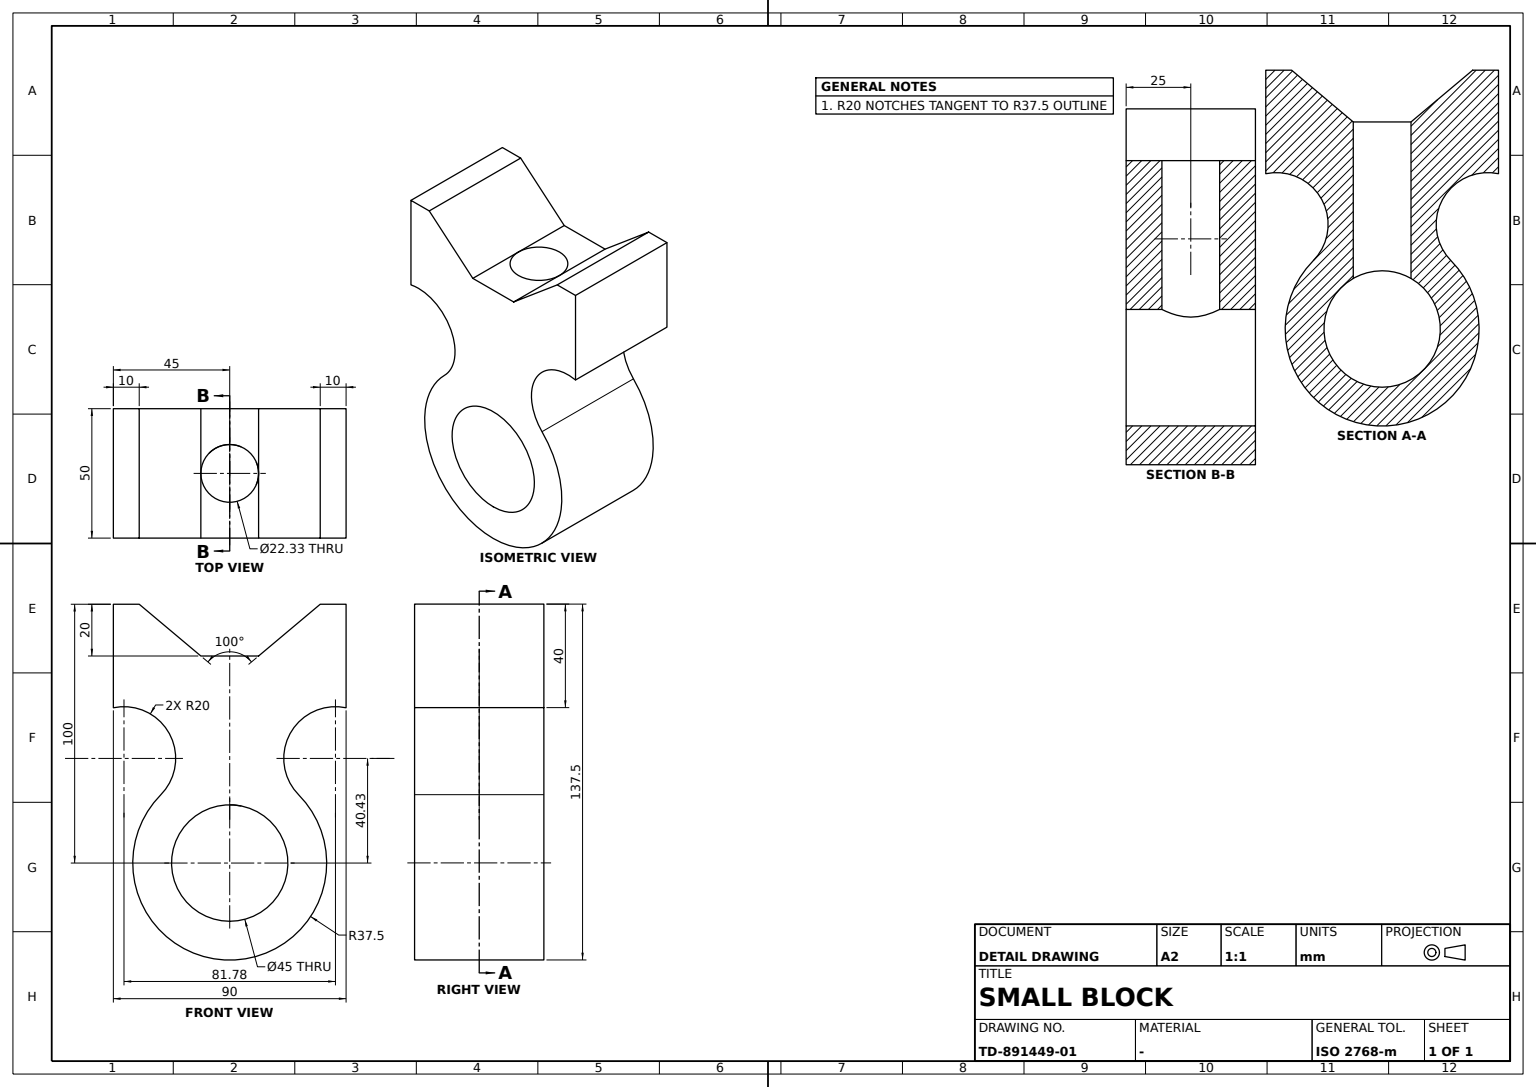
ISO-10303-21;
HEADER;
FILE_DESCRIPTION((''),'2;1');
FILE_NAME('','',(''),(''),'','','');
FILE_SCHEMA(('AUTOMOTIVE_DESIGN'));
ENDSEC;
DATA;
#1=APPLICATION_CONTEXT('');
#2=PRODUCT_CONTEXT('',#1,'mechanical');
#3=PRODUCT('','','',(#2));
#4=PRODUCT_DEFINITION_FORMATION('','',#3);
#5=PRODUCT_DEFINITION_CONTEXT('',#1,'design');
#6=PRODUCT_DEFINITION('','',#4,#5);
#7=PRODUCT_DEFINITION_SHAPE('','',#6);
#8=(LENGTH_UNIT()NAMED_UNIT(*)SI_UNIT(.MILLI.,.METRE.));
#9=(NAMED_UNIT(*)PLANE_ANGLE_UNIT()SI_UNIT($,.RADIAN.));
#10=(NAMED_UNIT(*)SI_UNIT($,.STERADIAN.)SOLID_ANGLE_UNIT());
#11=UNCERTAINTY_MEASURE_WITH_UNIT(LENGTH_MEASURE(0.005),#8,'distance_accuracy_value','');
#12=(GEOMETRIC_REPRESENTATION_CONTEXT(3)GLOBAL_UNCERTAINTY_ASSIGNED_CONTEXT((#11))GLOBAL_UNIT_ASSIGNED_CONTEXT((#8,#9,#10))REPRESENTATION_CONTEXT('',''));
#13=CARTESIAN_POINT('',(0.,-11.164928,80.));
#14=VERTEX_POINT('',#13);
#15=CARTESIAN_POINT('',(0.,11.164928,80.));
#16=VERTEX_POINT('',#15);
#17=CARTESIAN_POINT('',(0.,0.,80.));
#18=DIRECTION('',(0.,0.,-1.));
#19=DIRECTION('',(-1.,0.,0.));
#20=AXIS2_PLACEMENT_3D('',#17,#18,#19);
#21=CIRCLE('',#20,11.164928);
#22=EDGE_CURVE('',#14,#16,#21,.F.);
#23=ORIENTED_EDGE('',*,*,#22,.F.);
#24=CARTESIAN_POINT('',(25.,-11.164928,80.));
#25=VERTEX_POINT('',#24);
#26=DIRECTION('',(1.,0.,0.));
#27=VECTOR('',#26,1000.);
#28=LINE('',#13,#27);
#29=EDGE_CURVE('',#14,#25,#28,.T.);
#30=ORIENTED_EDGE('',*,*,#29,.T.);
#31=CARTESIAN_POINT('',(25.,11.164928,80.));
#32=VERTEX_POINT('',#31);
#33=CARTESIAN_POINT('',(25.,0.,80.));
#34=DIRECTION('',(0.,1.,0.));
#35=VECTOR('',#34,1000.);
#36=LINE('',#33,#35);
#37=EDGE_CURVE('',#25,#32,#36,.T.);
#38=ORIENTED_EDGE('',*,*,#37,.T.);
#39=LINE('',#15,#27);
#40=EDGE_CURVE('',#16,#32,#39,.T.);
#41=ORIENTED_EDGE('',*,*,#40,.F.);
#42=EDGE_LOOP('',(#23,#30,#38,#41));
#43=FACE_BOUND('',#42,.T.);
#44=AXIS2_PLACEMENT_3D('',#13,#18,#34);
#45=PLANE('',#44);
#46=ADVANCED_FACE('',(#43),#45,.F.);
#47=CARTESIAN_POINT('',(25.,-45.,100.));
#48=VERTEX_POINT('',#47);
#49=CARTESIAN_POINT('',(25.,-35.,100.));
#50=VERTEX_POINT('',#49);
#51=CARTESIAN_POINT('',(25.,0.,100.));
#52=LINE('',#51,#35);
#53=EDGE_CURVE('',#48,#50,#52,.T.);
#54=ORIENTED_EDGE('',*,*,#53,.T.);
#55=CARTESIAN_POINT('',(-25.,-35.,100.));
#56=VERTEX_POINT('',#55);
#57=CARTESIAN_POINT('',(0.,-35.,100.));
#58=LINE('',#57,#27);
#59=EDGE_CURVE('',#56,#50,#58,.T.);
#60=ORIENTED_EDGE('',*,*,#59,.F.);
#61=CARTESIAN_POINT('',(-25.,-45.,100.));
#62=VERTEX_POINT('',#61);
#63=CARTESIAN_POINT('',(-25.,0.,100.));
#64=LINE('',#63,#35);
#65=EDGE_CURVE('',#62,#56,#64,.T.);
#66=ORIENTED_EDGE('',*,*,#65,.F.);
#67=CARTESIAN_POINT('',(0.,-45.,100.));
#68=LINE('',#67,#27);
#69=EDGE_CURVE('',#62,#48,#68,.T.);
#70=ORIENTED_EDGE('',*,*,#69,.T.);
#71=EDGE_LOOP('',(#54,#60,#66,#70));
#72=FACE_BOUND('',#71,.T.);
#73=CARTESIAN_POINT('',(0.,35.,100.));
#74=AXIS2_PLACEMENT_3D('',#73,#18,#34);
#75=PLANE('',#74);
#76=ADVANCED_FACE('',(#72),#75,.F.);
#77=CARTESIAN_POINT('',(-25.,35.,100.));
#78=VERTEX_POINT('',#77);
#79=CARTESIAN_POINT('',(25.,35.,100.));
#80=VERTEX_POINT('',#79);
#81=LINE('',#73,#27);
#82=EDGE_CURVE('',#78,#80,#81,.T.);
#83=ORIENTED_EDGE('',*,*,#82,.F.);
#84=CARTESIAN_POINT('',(-25.,11.164928,80.));
#85=VERTEX_POINT('',#84);
#86=CARTESIAN_POINT('',(-25.,-34.779231,41.448273));
#87=DIRECTION('',(0.,0.766044443,0.64278761));
#88=VECTOR('',#87,1000.);
#89=LINE('',#86,#88);
#90=EDGE_CURVE('',#85,#78,#89,.T.);
#91=ORIENTED_EDGE('',*,*,#90,.F.);
#92=EDGE_CURVE('',#85,#16,#39,.T.);
#93=ORIENTED_EDGE('',*,*,#92,.T.);
#94=ORIENTED_EDGE('',*,*,#40,.T.);
#95=CARTESIAN_POINT('',(25.,-34.779231,41.448273));
#96=LINE('',#95,#88);
#97=EDGE_CURVE('',#32,#80,#96,.T.);
#98=ORIENTED_EDGE('',*,*,#97,.T.);
#99=EDGE_LOOP('',(#83,#91,#93,#94,#98));
#100=FACE_BOUND('',#99,.T.);
#101=DIRECTION('',(0.,0.64278761,-0.766044443));
#102=AXIS2_PLACEMENT_3D('',#15,#101,#87);
#103=PLANE('',#102);
#104=ADVANCED_FACE('',(#100),#103,.F.);
#105=CARTESIAN_POINT('',(-25.,0.,-22.5));
#106=VERTEX_POINT('',#105);
#107=CARTESIAN_POINT('',(-25.,0.,0.));
#108=AXIS2_PLACEMENT_3D('',#107,#26,#18);
#109=CIRCLE('',#108,22.5);
#110=EDGE_CURVE('',#106,#106,#109,.T.);
#111=ORIENTED_EDGE('',*,*,#110,.T.);
#112=EDGE_LOOP('',(#111));
#113=FACE_BOUND('',#112,.T.);
#114=ORIENTED_EDGE('',*,*,#90,.T.);
#115=CARTESIAN_POINT('',(-25.,45.,100.));
#116=VERTEX_POINT('',#115);
#117=EDGE_CURVE('',#78,#116,#64,.T.);
#118=ORIENTED_EDGE('',*,*,#117,.T.);
#119=CARTESIAN_POINT('',(-25.,45.,60.));
#120=VERTEX_POINT('',#119);
#121=CARTESIAN_POINT('',(-25.,45.,0.));
#122=VECTOR('',#18,1000.);
#123=LINE('',#121,#122);
#124=EDGE_CURVE('',#116,#120,#123,.T.);
#125=ORIENTED_EDGE('',*,*,#124,.T.);
#126=CARTESIAN_POINT('',(-25.,26.666657,26.365496));
#127=VERTEX_POINT('',#126);
#128=CARTESIAN_POINT('',(-25.,40.888875,40.427094));
#129=AXIS2_PLACEMENT_3D('',#128,#26,#18);
#130=CIRCLE('',#129,20.);
#131=EDGE_CURVE('',#120,#127,#130,.T.);
#132=ORIENTED_EDGE('',*,*,#131,.T.);
#133=CARTESIAN_POINT('',(-25.,-26.666657,26.365496));
#134=VERTEX_POINT('',#133);
#135=CIRCLE('',#108,37.5);
#136=EDGE_CURVE('',#134,#127,#135,.T.);
#137=ORIENTED_EDGE('',*,*,#136,.F.);
#138=CARTESIAN_POINT('',(-25.,-45.,60.));
#139=VERTEX_POINT('',#138);
#140=CARTESIAN_POINT('',(-25.,-40.888875,40.427094));
#141=AXIS2_PLACEMENT_3D('',#140,#26,#18);
#142=CIRCLE('',#141,20.);
#143=EDGE_CURVE('',#134,#139,#142,.T.);
#144=ORIENTED_EDGE('',*,*,#143,.T.);
#145=CARTESIAN_POINT('',(-25.,-45.,0.));
#146=DIRECTION('',(0.,0.,1.));
#147=VECTOR('',#146,1000.);
#148=LINE('',#145,#147);
#149=EDGE_CURVE('',#139,#62,#148,.T.);
#150=ORIENTED_EDGE('',*,*,#149,.T.);
#151=ORIENTED_EDGE('',*,*,#65,.T.);
#152=CARTESIAN_POINT('',(-25.,-11.164928,80.));
#153=VERTEX_POINT('',#152);
#154=CARTESIAN_POINT('',(-25.,34.779231,41.448273));
#155=DIRECTION('',(0.,0.766044443,-0.64278761));
#156=VECTOR('',#155,1000.);
#157=LINE('',#154,#156);
#158=EDGE_CURVE('',#56,#153,#157,.T.);
#159=ORIENTED_EDGE('',*,*,#158,.T.);
#160=CARTESIAN_POINT('',(-25.,0.,80.));
#161=LINE('',#160,#35);
#162=EDGE_CURVE('',#153,#85,#161,.T.);
#163=ORIENTED_EDGE('',*,*,#162,.T.);
#164=EDGE_LOOP('',(#114,#118,#125,#132,#137,#144,#150,#151,#159,#163));
#165=FACE_BOUND('',#164,.T.);
#166=AXIS2_PLACEMENT_3D('',#107,#26,#34);
#167=PLANE('',#166);
#168=ADVANCED_FACE('',(#113,#165),#167,.F.);
#169=CARTESIAN_POINT('',(25.,34.779231,41.448273));
#170=LINE('',#169,#156);
#171=EDGE_CURVE('',#50,#25,#170,.T.);
#172=ORIENTED_EDGE('',*,*,#171,.T.);
#173=ORIENTED_EDGE('',*,*,#29,.F.);
#174=EDGE_CURVE('',#153,#14,#28,.T.);
#175=ORIENTED_EDGE('',*,*,#174,.F.);
#176=ORIENTED_EDGE('',*,*,#158,.F.);
#177=ORIENTED_EDGE('',*,*,#59,.T.);
#178=EDGE_LOOP('',(#172,#173,#175,#176,#177));
#179=FACE_BOUND('',#178,.T.);
#180=DIRECTION('',(0.,-0.64278761,-0.766044443));
#181=AXIS2_PLACEMENT_3D('',#57,#180,#155);
#182=PLANE('',#181);
#183=ADVANCED_FACE('',(#179),#182,.F.);
#184=CARTESIAN_POINT('',(25.,0.,-22.5));
#185=VERTEX_POINT('',#184);
#186=CARTESIAN_POINT('',(25.,0.,0.));
#187=AXIS2_PLACEMENT_3D('',#186,#26,#18);
#188=CIRCLE('',#187,22.5);
#189=EDGE_CURVE('',#185,#185,#188,.T.);
#190=ORIENTED_EDGE('',*,*,#189,.T.);
#191=EDGE_LOOP('',(#190));
#192=FACE_BOUND('',#191,.T.);
#193=ORIENTED_EDGE('',*,*,#110,.F.);
#194=EDGE_LOOP('',(#193));
#195=FACE_BOUND('',#194,.T.);
#196=CARTESIAN_POINT('',(-11.164928,0.,22.5));
#197=VERTEX_POINT('',#196);
#198=CARTESIAN_POINT('',(-10.549112,4.471728,22.185581));
#199=CARTESIAN_POINT('',(-11.471357,-0.004788,22.656475));
#200=CARTESIAN_POINT('',(-10.555027,-4.452577,22.188517));
#201=CARTESIAN_POINT('',(-8.083695,-8.096902,21.079337));
#202=CARTESIAN_POINT('',(-4.460245,-10.54731,19.903886));
#203=CARTESIAN_POINT('',(-0.033968,-11.469433,19.351981));
#204=CARTESIAN_POINT('',(4.433612,-10.564331,19.894948));
#205=CARTESIAN_POINT('',(8.071653,-8.106887,21.074896));
#206=CARTESIAN_POINT('',(10.544117,-4.481106,22.183139));
#207=CARTESIAN_POINT('',(11.471336,-0.0131,22.656464));
#208=CARTESIAN_POINT('',(10.560049,4.443068,22.190975));
#209=CARTESIAN_POINT('',(8.089148,8.091903,21.081417));
#210=CARTESIAN_POINT('',(4.463912,10.546318,19.904537));
#211=CARTESIAN_POINT('',(0.033992,11.469928,19.351655));
#212=CARTESIAN_POINT('',(-4.437338,10.56334,19.895601));
#213=CARTESIAN_POINT('',(-8.077104,8.101877,21.076977));
#214=B_SPLINE_CURVE_WITH_KNOTS('',3,(#198,#199,#200,#201,#202,#203,#204,#205,#206,#207,#208,#209,#210,#211,#212,#213,#198,#199,#200),.UNSPECIFIED.,.T.,.F.,(1,1,1,1,1,1,1,1,1,1,1,1,1,1,1,1,1,1,1,1,1,1,1),(-0.013302099,-0.008868066,-0.004434033,0.,0.004434033,0.008868066,0.013302099,0.017736132,0.022170165,0.026604198,0.031038231,0.035472264,0.039906297,0.04434033,0.048774363,0.053208396,0.057642429,0.062076462,0.066510495,0.070944528,0.075378561,0.079812594,0.084246628),.UNSPECIFIED.);
#215=EDGE_CURVE('',#197,#197,#214,.T.);
#216=ORIENTED_EDGE('',*,*,#215,.T.);
#217=EDGE_LOOP('',(#216));
#218=FACE_BOUND('',#217,.T.);
#219=CARTESIAN_POINT('',(0.,0.,0.));
#220=AXIS2_PLACEMENT_3D('',#219,#26,#34);
#221=CYLINDRICAL_SURFACE('',#220,22.5);
#222=ADVANCED_FACE('',(#192,#195,#218),#221,.F.);
#223=ORIENTED_EDGE('',*,*,#215,.F.);
#224=EDGE_LOOP('',(#223));
#225=FACE_BOUND('',#224,.T.);
#226=ORIENTED_EDGE('',*,*,#22,.T.);
#227=EDGE_CURVE('',#16,#14,#21,.F.);
#228=ORIENTED_EDGE('',*,*,#227,.T.);
#229=EDGE_LOOP('',(#226,#228));
#230=FACE_BOUND('',#229,.T.);
#231=CARTESIAN_POINT('',(0.,0.,20.59));
#232=AXIS2_PLACEMENT_3D('',#231,#146,#26);
#233=CYLINDRICAL_SURFACE('',#232,11.164928);
#234=ADVANCED_FACE('',(#225,#230),#233,.F.);
#235=ORIENTED_EDGE('',*,*,#117,.F.);
#236=ORIENTED_EDGE('',*,*,#82,.T.);
#237=CARTESIAN_POINT('',(25.,45.,100.));
#238=VERTEX_POINT('',#237);
#239=EDGE_CURVE('',#80,#238,#52,.T.);
#240=ORIENTED_EDGE('',*,*,#239,.T.);
#241=CARTESIAN_POINT('',(0.,45.,100.));
#242=LINE('',#241,#27);
#243=EDGE_CURVE('',#116,#238,#242,.T.);
#244=ORIENTED_EDGE('',*,*,#243,.F.);
#245=EDGE_LOOP('',(#235,#236,#240,#244));
#246=FACE_BOUND('',#245,.T.);
#247=ADVANCED_FACE('',(#246),#75,.F.);
#248=CARTESIAN_POINT('',(25.,45.,60.));
#249=VERTEX_POINT('',#248);
#250=LINE('',#119,#27);
#251=EDGE_CURVE('',#120,#249,#250,.T.);
#252=ORIENTED_EDGE('',*,*,#251,.T.);
#253=CARTESIAN_POINT('',(25.,26.666657,26.365496));
#254=VERTEX_POINT('',#253);
#255=CARTESIAN_POINT('',(25.,40.888875,40.427094));
#256=AXIS2_PLACEMENT_3D('',#255,#26,#18);
#257=CIRCLE('',#256,20.);
#258=EDGE_CURVE('',#249,#254,#257,.T.);
#259=ORIENTED_EDGE('',*,*,#258,.T.);
#260=CARTESIAN_POINT('',(0.,26.666657,26.365496));
#261=LINE('',#260,#27);
#262=EDGE_CURVE('',#127,#254,#261,.T.);
#263=ORIENTED_EDGE('',*,*,#262,.F.);
#264=ORIENTED_EDGE('',*,*,#131,.F.);
#265=EDGE_LOOP('',(#252,#259,#263,#264));
#266=FACE_BOUND('',#265,.T.);
#267=CARTESIAN_POINT('',(0.,40.888875,40.427094));
#268=AXIS2_PLACEMENT_3D('',#267,#26,#34);
#269=CYLINDRICAL_SURFACE('',#268,20.);
#270=ADVANCED_FACE('',(#266),#269,.F.);
#271=CARTESIAN_POINT('',(25.,-45.,60.));
#272=VERTEX_POINT('',#271);
#273=LINE('',#138,#27);
#274=EDGE_CURVE('',#139,#272,#273,.T.);
#275=ORIENTED_EDGE('',*,*,#274,.T.);
#276=CARTESIAN_POINT('',(25.,-45.,0.));
#277=LINE('',#276,#147);
#278=EDGE_CURVE('',#272,#48,#277,.T.);
#279=ORIENTED_EDGE('',*,*,#278,.T.);
#280=ORIENTED_EDGE('',*,*,#69,.F.);
#281=ORIENTED_EDGE('',*,*,#149,.F.);
#282=EDGE_LOOP('',(#275,#279,#280,#281));
#283=FACE_BOUND('',#282,.T.);
#284=CARTESIAN_POINT('',(0.,-45.,60.));
#285=AXIS2_PLACEMENT_3D('',#284,#34,#146);
#286=PLANE('',#285);
#287=ADVANCED_FACE('',(#283),#286,.F.);
#288=ORIENTED_EDGE('',*,*,#136,.T.);
#289=ORIENTED_EDGE('',*,*,#262,.T.);
#290=CARTESIAN_POINT('',(25.,-26.666657,26.365496));
#291=VERTEX_POINT('',#290);
#292=CIRCLE('',#187,37.5);
#293=EDGE_CURVE('',#291,#254,#292,.T.);
#294=ORIENTED_EDGE('',*,*,#293,.F.);
#295=CARTESIAN_POINT('',(0.,-26.666657,26.365496));
#296=LINE('',#295,#27);
#297=EDGE_CURVE('',#134,#291,#296,.T.);
#298=ORIENTED_EDGE('',*,*,#297,.F.);
#299=EDGE_LOOP('',(#288,#289,#294,#298));
#300=FACE_BOUND('',#299,.T.);
#301=CYLINDRICAL_SURFACE('',#220,37.5);
#302=ADVANCED_FACE('',(#300),#301,.T.);
#303=ORIENTED_EDGE('',*,*,#293,.T.);
#304=ORIENTED_EDGE('',*,*,#258,.F.);
#305=CARTESIAN_POINT('',(25.,45.,0.));
#306=LINE('',#305,#122);
#307=EDGE_CURVE('',#238,#249,#306,.T.);
#308=ORIENTED_EDGE('',*,*,#307,.F.);
#309=ORIENTED_EDGE('',*,*,#239,.F.);
#310=ORIENTED_EDGE('',*,*,#97,.F.);
#311=ORIENTED_EDGE('',*,*,#37,.F.);
#312=ORIENTED_EDGE('',*,*,#171,.F.);
#313=ORIENTED_EDGE('',*,*,#53,.F.);
#314=ORIENTED_EDGE('',*,*,#278,.F.);
#315=CARTESIAN_POINT('',(25.,-40.888875,40.427094));
#316=AXIS2_PLACEMENT_3D('',#315,#26,#18);
#317=CIRCLE('',#316,20.);
#318=EDGE_CURVE('',#291,#272,#317,.T.);
#319=ORIENTED_EDGE('',*,*,#318,.F.);
#320=EDGE_LOOP('',(#303,#304,#308,#309,#310,#311,#312,#313,#314,#319));
#321=FACE_BOUND('',#320,.T.);
#322=ORIENTED_EDGE('',*,*,#189,.F.);
#323=EDGE_LOOP('',(#322));
#324=FACE_BOUND('',#323,.T.);
#325=AXIS2_PLACEMENT_3D('',#186,#26,#34);
#326=PLANE('',#325);
#327=ADVANCED_FACE('',(#321,#324),#326,.T.);
#328=ORIENTED_EDGE('',*,*,#227,.F.);
#329=ORIENTED_EDGE('',*,*,#92,.F.);
#330=ORIENTED_EDGE('',*,*,#162,.F.);
#331=ORIENTED_EDGE('',*,*,#174,.T.);
#332=EDGE_LOOP('',(#328,#329,#330,#331));
#333=FACE_BOUND('',#332,.T.);
#334=ADVANCED_FACE('',(#333),#45,.F.);
#335=ORIENTED_EDGE('',*,*,#307,.T.);
#336=ORIENTED_EDGE('',*,*,#251,.F.);
#337=ORIENTED_EDGE('',*,*,#124,.F.);
#338=ORIENTED_EDGE('',*,*,#243,.T.);
#339=EDGE_LOOP('',(#335,#336,#337,#338));
#340=FACE_BOUND('',#339,.T.);
#341=DIRECTION('',(0.,-1.,0.));
#342=AXIS2_PLACEMENT_3D('',#241,#341,#18);
#343=PLANE('',#342);
#344=ADVANCED_FACE('',(#340),#343,.F.);
#345=ORIENTED_EDGE('',*,*,#318,.T.);
#346=ORIENTED_EDGE('',*,*,#274,.F.);
#347=ORIENTED_EDGE('',*,*,#143,.F.);
#348=ORIENTED_EDGE('',*,*,#297,.T.);
#349=EDGE_LOOP('',(#345,#346,#347,#348));
#350=FACE_BOUND('',#349,.T.);
#351=CARTESIAN_POINT('',(0.,-40.888875,40.427094));
#352=AXIS2_PLACEMENT_3D('',#351,#26,#34);
#353=CYLINDRICAL_SURFACE('',#352,20.);
#354=ADVANCED_FACE('',(#350),#353,.F.);
#355=CLOSED_SHELL('',(#46,#76,#104,#168,#183,#222,#234,#247,#270,#287,#302,#327,#334,#344,#354));
#356=MANIFOLD_SOLID_BREP('',#355);
#357=ADVANCED_BREP_SHAPE_REPRESENTATION('',(#356),#12);
#358=SHAPE_DEFINITION_REPRESENTATION(#7,#357);
ENDSEC;
END-ISO-10303-21;
